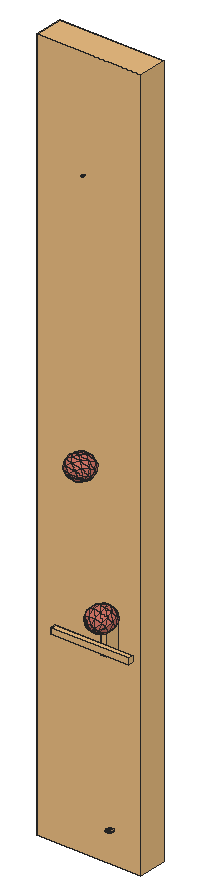
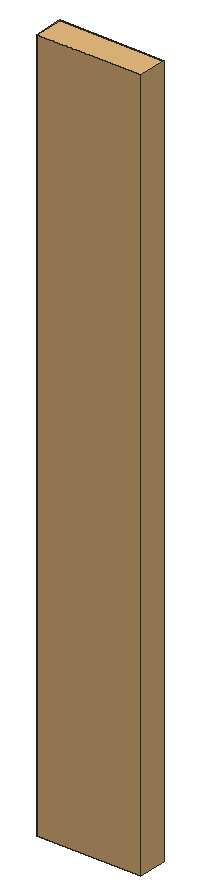
# SketchUp Ruby script. Lengths in inches.
U = 1.inch
M = Sketchup.active_model
def pt(a) = Geom::Point3d.new(a.map { |v| v * U })
def face(e, loops, mat)
  f = e.add_face(loops[0].map { |a| pt(a) })
  loops[1..].each { |l| e.add_face(l.map { |a| pt(a) }).erase! }
  f.material = f.back_material = mat if mat
  f
end
# faces: each face lists its corners as indices into pts; further lists are holes
def faces(e, pts, list, mat = nil) = list.each { |f| face(e, (f[0].is_a?(Array) ? f : [f]).map { |l| l.map { |i| pts[i] } }, mat) }
# xy, xz, yz: faces in a plane at the given z, y or x. An outline is a flat list of corners, or four numbers for a rectangle; further outlines are holes
def ring(l) = l.size == 4 ? [[l[0], l[1]], [l[2], l[1]], [l[2], l[3]], [l[0], l[3]]] : l.each_slice(2).to_a
def flat(e, list, mat, &to3) = list.each { |f| face(e, (f[0].is_a?(Array) ? f : [f]).map { |l| ring(l).map { |u, v| to3.(u, v) } }, mat) }
def xy(e, z, list, mat = nil) = flat(e, list, mat) { |x, y| [x, y, z] }
def xz(e, y, list, mat = nil) = flat(e, list, mat) { |x, z| [x, y, z] }
def yz(e, x, list, mat = nil) = flat(e, list, mat) { |y, z| [x, y, z] }
def lines(e, pts, list) = list.each { |a, b| e.add_line(pt(pts[a]), pt(pts[b])) }
# prism: a flat outline (further loops are holes) pulled along v
def prism(e, loops, v, mat = nil)
  f = face(e, loops, mat); d = Geom::Vector3d.new(v.map { |x| x * U })
  f.pushpull(f.normal.samedirection?(d) ? d.length : -d.length)
end
def box(e, o, s, mat = nil) = prism(e, [[o, [o[0] + s[0], o[1], o[2]], [o[0] + s[0], o[1] + s[1], o[2]], [o[0], o[1] + s[1], o[2]]]], [0, 0, s[2]], mat)
def at(x, y, z, deg = 0) = Geom::Transformation.translation(pt([x, y, z])) * Geom::Transformation.rotation(ORIGIN, Z_AXIS, deg.degrees)
def axes(o, x, y, z) = Geom::Transformation.new([*x, 0, *y, 0, *z, 0, *pt(o).to_a, 1])
def part(name) = M.definitions.add(name)
# library, detail: a bought-in or finely detailed component or shape, given as its bounding box
def library(name, o, s) = part(name).tap { |d| box(d.entities, o, s) }
def detail(e, o, s) = box(e.add_group.entities, o, s)
def put(e, d, t, mat = nil) = e.add_instance(d, t).tap { |i| i.material = mat if mat }
def group(e, t, mat = nil) = e.add_group.tap { |g| g.transformation = t; g.material = mat if mat }.entities
root = M.entities
M.materials.add("green").color = [174, 139, 102]
M.materials.add("vio").color = [206, 114, 100]
c1 = part("3DGeom~237_Defintion")
p = [[47.04,-55.62,-493.71],[-13.56,-317.59,-331.8],[-140.27,-151.99,-445.55],[202.73,-206.32,-387.4],[187.3,88.625,-451.96],[-121.25,109.98,-467.72],
  [-40.27,193.26,-443.62],[-229.4,54.34,-439.92],[-257.06,246.11,-316.41],[364.69,-39.76,-339.2],[242.94,242.09,-331.5],[-8.15,281.87,-374.07],
  [-226.21,-343.77,-187.29],[-324.43,-174.66,-320.41],[-335.72,41.26,-367.67],[202.73,-206.32,-387.4],[116.79,-398.1,-129.14],[-13.56,-317.59,-331.8],
  [202.73,-206.32,-387.4],[304.09,-301.74,-177.3],[364.69,-39.76,-339.2],[304.09,-301.74,-177.3],[202.73,-206.32,-387.4],[-33.49,352.06,-277.72],
  [242.94,242.09,-331.5],[-8.15,281.87,-374.07],[-33.49,352.06,-277.72],[-335.72,41.26,-367.67],[-324.43,-174.66,-320.41],[-456.1,-117.56,-151.8],
  [-335.72,41.26,-367.67],[-411.74,74.22,-270.32],[-335.72,41.26,-367.67],[-257.06,246.11,-316.41],[364.69,-39.76,-339.2],[444.36,-157.49,-135.55],
  [304.09,-301.74,-177.3],[428.9375,137.45,-200.11],[364.69,-39.76,-339.2],[428.9375,137.45,-200.11],[-13.56,-317.59,-331.8],[-67.38,-420.77,-4],
  [-226.21,-343.77,-187.29],[-13.56,-317.59,-331.8],[199.05,363.67,-164.61],[428.9375,137.45,-200.11],[242.94,242.09,-331.5],[-33.49,352.06,-277.72],
  [199.05,363.67,-164.61],[242.94,242.09,-331.5],[-324.43,-174.66,-320.41],[-226.21,-343.77,-187.29],[-378.25,-277.83,7.4],[-324.43,-174.66,-320.41],
  [-437.09,144.42,-173.96],[-257.06,246.11,-316.41],[-404.96,233.02,-104.42],[-257.06,246.11,-316.41],[-323.98,316.3,-80.32],[-257.06,246.11,-316.41],
  [-323.98,316.3,-80.32],[-215.84,371.9375,-108.12],[-257.06,246.11,-316.41],[-109.51,385.02,-180.37],[-33.49,352.06,-277.72],[-257.06,246.11,-316.41],
  [-257.06,246.11,-316.41],[-33.49,352.06,-277.72],[-500,4.02,15.09],[428.9375,137.45,-200.11],[500,-4.02,-15.09],[378.25,277.83,-7.4],
  [428.9375,137.45,-200.11],[199.05,363.67,-164.61],[428.9375,137.45,-200.11],[-226.21,-343.77,-187.29],[-199.05,-363.67,164.61],[-226.21,-343.77,-187.29],
  [-199.05,-363.67,164.61],[-378.25,-277.83,7.4],[67.38,420.77,4],[215.84,-371.9375,108.12],[323.98,-316.3,80.32],[323.98,-316.3,80.32],
  [304.09,-301.74,-177.3],[-444.36,157.49,135.55],[378.25,277.83,-7.4],[-428.9375,-137.45,200.11],[404.96,-233.02,104.42],[323.98,-316.3,80.32],
  [109.51,-385.02,180.37],[-116.78,398.1,129.14],[-304.09,301.73,177.3],[-304.09,301.73,177.3],[-323.98,316.3,-80.32],[-304.09,301.73,177.3],
  [437.09,-144.41,173.96],[456.1,117.56,151.8],[226.21,343.77,187.29],[226.21,343.77,187.29],[378.25,277.83,-7.4],[33.49,-352.06,277.72],
  [-199.05,-363.67,164.61],[-199.05,-363.67,164.61],[-242.94,-242.09,331.5],[-242.94,-242.09,331.5],[-364.69,39.76,339.2],[257.06,-246.11,316.41],
  [323.98,-316.3,80.32],[257.06,-246.11,316.41],[257.06,-246.11,316.41],[13.56,317.59,331.8],[-202.73,206.32,387.4],[-202.73,206.32,387.4],
  [-304.09,301.73,177.3],[411.74,-74.22,270.32],[324.43,174.66,320.41],[226.21,343.77,187.29],[-199.05,-363.67,164.61],[8.15,-281.86,374.07],
  [-242.94,-242.09,331.5],[-199.05,-363.67,164.61],[8.15,-281.86,374.07],[257.06,-246.11,316.41],[-202.73,206.32,387.4],[13.56,317.59,331.8],
  [324.43,174.66,320.41],[226.21,343.77,187.29],[-428.9375,-137.45,200.11],[-242.94,-242.09,331.5],[-187.3,-88.625,451.96],[-428.9375,-137.45,200.11],
  [-364.69,39.76,339.2],[335.72,-41.26,367.67],[257.06,-246.11,316.41],[8.15,-281.86,374.07],[33.49,-352.06,277.72],[257.06,-246.11,316.41],
  [40.27,-193.26,443.62],[257.06,-246.11,316.41],[121.25,-109.98,467.72],[257.06,-246.11,316.41],[229.4,-54.34,439.92],[257.06,-246.11,316.41],
  [335.72,-41.26,367.67],[257.06,-246.11,316.41],[140.27,151.99,445.55],[335.72,-41.26,367.67],[324.43,174.66,320.41],[13.56,317.59,331.8],
  [324.43,174.66,320.41],[-202.73,206.32,387.4],[13.56,317.59,331.8],[-364.69,39.76,339.2],[-47.04,55.62,493.71],[-364.69,39.76,339.2],
  [-202.73,206.32,387.4],[335.72,-41.26,367.67],[-202.73,206.32,387.4]]
faces(c1.entities,p,[[0,1,2],[0,3,1],[4,3,0],[5,0,2],[6,0,5],[6,4,0],[5,2,7],[5,7,8],
  [6,5,8],[4,9,3],[10,9,4],[11,4,6],[11,10,4],[2,12,13],[2,1,12],[7,2,13],
  [11,6,8],[7,13,14],[7,14,8],[15,16,17],[18,19,16],[20,21,22],[23,24,25],[26,11,8],
  [27,28,29],[30,29,31],[32,31,33],[34,35,36],[37,35,38],[10,39,9],[40,41,42],[43,16,41],
  [44,45,46],[47,48,49],[50,51,52],[53,52,29],[31,54,55],[54,56,57],[56,58,59],[60,61,62],
  [63,64,65],[61,63,66],[63,48,67],[31,29,68],[31,68,54],[69,70,35],[71,70,72],[73,71,74],
  [75,41,76],[77,78,79],[63,80,48],[61,80,63],[19,81,16],[19,82,81],[35,83,84],[54,68,85],
  [54,85,56],[80,86,48],[29,52,87],[29,87,68],[35,88,89],[70,88,35],[16,90,41],[16,81,90],
  [60,91,61],[61,91,80],[56,85,92],[56,93,94],[60,95,91],[70,96,88],[97,96,70],[71,97,70],
  [98,97,71],[80,99,100],[41,101,102],[41,90,101],[91,99,80],[52,103,104],[52,105,87],[68,87,106],
  [68,106,85],[81,82,107],[108,88,109],[88,96,110],[90,81,107],[95,111,91],[91,111,99],[85,106,112],
  [85,113,114],[97,115,96],[116,115,97],[117,116,97],[118,119,120],[121,101,122],[96,115,123],[95,124,111],
  [101,90,107],[125,126,127],[128,129,130],[131,130,132],[115,133,134],[116,133,115],[135,136,137],[138,135,139],
  [140,138,141],[142,140,143],[144,142,145],[146,147,148],[149,146,150],[129,135,138],[129,138,130],[151,146,152],
  [153,130,154],[155,154,156],[146,142,157],[158,154,146],[154,140,142],[154,142,146],[130,138,140],[130,140,154]],"vio")
c2 = library("3DGeom~136_Defintion",[-19.91,-529.75,-72.32],[39.82,1000,144.64])
c3 = part("3DGeom~46_Defintion")
p = [[-27.13,499.98,25.14],[-34.02,499.92,31.49],[-24.32,499.93,26.43],[-33.96,499.95,29.98],[-34.02,499.92,31.49],[-27.13,499.98,25.14],
  [-33.96,499.95,29.98],[-27.13,499.98,25.14],[-28.64,499.99,25.08],[-31.49,500,26.1],[-33.96,499.95,29.98],[-28.64,499.99,25.08],
  [-27.13,499.98,25.14],[-24.32,499.93,26.43],[-25.67,499.95,25.59],[-31.49,500,26.1],[-28.64,499.99,25.08],[-30.125,500,25.4],
  [-32.66,499.99,27.17],[-33.96,499.95,29.98],[-31.49,500,26.1],[-24.32,499.93,26.43],[-34.02,499.92,31.49],[-22.56,499.86,28.97],
  [-24.32,499.93,26.43],[-22.56,499.86,28.97],[-23.26,499.89,27.6],[-32.66,499.99,27.17],[-33.51,499.97,28.51],[-33.96,499.95,29.98],
  [-22.56,499.86,28.97],[-34.02,499.92,31.49],[-22.29,499.8,31.96],[-22.56,499.86,28.97],[-22.29,499.8,31.96],[-22.23,499.83,30.45],
  [-26.125,499.75,36.54],[-34.02,499.92,31.49],[-29.12,499.77,36.8],[-23.59,499.76,34.77],[-34.02,499.92,31.49],[-26.125,499.75,36.54],
  [-31.92,499.82,35.51],[-34.02,499.92,31.49],[-33.69,499.89,32.97],[-29.12,499.77,36.8],[-34.02,499.92,31.49],[-31.92,499.82,35.51],
  [-22.29,499.8,31.96],[-34.02,499.92,31.49],[-23.59,499.76,34.77],[-22.29,499.8,31.96],[-23.59,499.76,34.77],[-22.74,499.78,33.43],
  [-31.92,499.82,35.51],[-33.69,499.89,32.97],[-32.99,499.85,34.33],[-23.59,499.76,34.77],[-26.125,499.75,36.54],[-24.76,499.75,35.84],
  [-29.12,499.77,36.8],[-31.92,499.82,35.51],[-30.58,499.79,36.35],[-26.125,499.75,36.54],[-29.12,499.77,36.8],[-27.6,499.76,36.86],
  [-53.29,-499.72,58.02],[-51.39,-499.92,55.77],[-50.77,-499.95,55.72],[-53.29,-499.72,58.02],[-50.77,-499.95,55.72],[-53.24,-499.7,58.64],
  [-50.77,-499.95,55.72],[-49.57,-500,56.11],[-53.24,-499.7,58.64],[-50.77,-499.95,55.72],[-50.16,-499.98,55.83],[-49.57,-500,56.11],
  [-52.49,-499.84,56.33],[-51.39,-499.92,55.77],[-53.29,-499.72,58.02],[-52.49,-499.84,56.33],[-51.97,-499.88,55.98],[-51.39,-499.92,55.77],
  [-49.57,-500,56.11],[-48.72,-499.99,57.04],[-53.24,-499.7,58.64],[-49.57,-500,56.11],[-49.08,-500,56.53],[-48.72,-499.99,57.04],
  [-53.29,-499.72,58.02],[-52.91,-499.8,56.82],[-52.49,-499.84,56.33],[-53.29,-499.72,58.02],[-53.18,-499.76,57.41],[-52.91,-499.8,56.82],
  [-48.72,-499.99,57.04],[-48.46,-499.95,58.24],[-53.24,-499.7,58.64],[-48.72,-499.99,57.04],[-48.52,-499.98,57.63],[-48.46,-499.95,58.24],
  [-48.46,-499.95,58.24],[-48.85,-499.875,59.45],[-53.24,-499.7,58.64],[-48.46,-499.95,58.24],[-48.57,-499.91,58.86],[-48.85,-499.875,59.45],
  [-48.85,-499.875,59.45],[-49.78,-499.79,60.29],[-53.24,-499.7,58.64],[-49.78,-499.79,60.29],[-50.98,-499.72,60.54],[-53.24,-499.7,58.64],
  [-52.18,-499.68,60.16],[-53.03,-499.68,59.22],[-53.24,-499.7,58.64],[-50.98,-499.72,60.54],[-52.18,-499.68,60.16],[-53.24,-499.7,58.64],
  [-52.18,-499.68,60.16],[-52.68,-499.67,59.74],[-53.03,-499.68,59.22],[-48.85,-499.875,59.45],[-49.26,-499.83,59.9375],[-49.78,-499.79,60.29],
  [-50.98,-499.72,60.54],[-51.6,-499.69,60.4375],[-52.18,-499.68,60.16],[-49.78,-499.79,60.29],[-50.36,-499.75,60.49],[-50.98,-499.72,60.54]]
faces(c3.entities,p,[[0,1,2],[3,4,5],[6,7,8],[9,10,11],[12,13,14],[15,16,17],[18,19,20],[21,22,23],
  [24,25,26],[27,28,29],[30,31,32],[33,34,35],[36,37,38],[39,40,41],[42,43,44],[45,46,47],
  [48,49,50],[51,52,53],[54,55,56],[57,58,59],[60,61,62],[63,64,65],[66,67,68],[69,70,71],
  [72,73,74],[75,76,77],[78,79,80],[81,82,83],[84,85,86],[87,88,89],[90,91,92],[93,94,95],
  [96,97,98],[99,100,101],[102,103,104],[105,106,107],[108,109,110],[111,112,113],[114,115,116],[117,118,119],
  [120,121,122],[123,124,125],[126,127,128],[129,130,131]],"green")
c4 = library("3DGeom~169_Defintion",[-36.08,-38.12,-500],[72.16,76.24,1000])
c5 = part("3DGeom~170_Defintion")
p = [[22.63,21.29,-499.8],[10.94,15.58,-499.92],[15.89,19.76,-500],[22.63,21.29,-499.8],[9.12,9.86,-499.6],[10.94,15.58,-499.92],
  [22.63,21.29,-499.8],[22.56,-1.57,-498.16],[15.83,-0.04,-498.58],[22.63,21.29,-499.8],[29.3,-0.04,-497.96],[22.56,-1.57,-498.16],
  [22.63,21.29,-499.8],[15.83,-0.04,-498.58],[10.91,4.15,-499.1],[22.63,21.29,-499.8],[34.25,4.15,-498.04],[29.3,-0.04,-497.96],
  [22.63,21.29,-499.8],[10.91,4.15,-499.1],[9.12,9.86,-499.6],[22.63,21.29,-499.8],[36.08,9.86,-498.37],[34.25,4.15,-498.04],
  [22.63,21.29,-499.8],[34.29,15.58,-498.86],[36.08,9.86,-498.37],[22.63,21.29,-499.8],[29.37,19.76,-499.39],[34.29,15.58,-498.86],
  [-22.3,-38.12,487.14],[-22.89,-17.99,500],[-34.125,-33.09,489.82],[-22.3,-38.12,487.14],[-34.125,-33.09,489.82],[-29.08,-36.77,487.69],
  [-10.78,-33.09,490.89],[-22.89,-17.99,500],[-22.3,-38.12,487.14],[-10.78,-33.09,490.89],[-22.3,-38.12,487.14],[-15.6,-36.77,488.31],
  [-34.125,-33.09,489.82],[-34.42,-23.02,496.25],[-36.08,-28.06,492.96],[-34.125,-33.09,489.82],[-22.89,-17.99,500],[-34.42,-23.02,496.25],
  [-11.07,-23.02,497.32],[-22.89,-17.99,500],[-10.78,-33.09,490.89],[-11.07,-23.02,497.32],[-10.78,-33.09,490.89],[-9.12,-28.06,494.18],
  [-22.89,-17.99,500],[-29.59,-19.34,498.83],[-34.42,-23.02,496.25],[-22.89,-17.99,500],[-11.07,-23.02,497.32],[-16.11,-19.34,499.45]]
faces(c5.entities,p,[[0,1,2],[3,4,5],[6,7,8],[9,10,11],[12,13,14],[15,16,17],[18,19,20],[21,22,23],
  [24,25,26],[27,28,29],[30,31,32],[33,34,35],[36,37,38],[39,40,41],[42,43,44],[45,46,47],
  [48,49,50],[51,52,53],[54,55,56],[57,58,59]],"green")
c6 = part("3DGeom~233_Defintion")
p = [[65.95,-313.47,-334.33],[-179.28,-246.09,-369.2],[-76.8125,-70.73,-489.54],[154.6875,-161.61,-438.54],[-287.73,39.11,-409.37],[46.24,123.59,-478.71],
  [-181.17,207.39,-399.98],[261.25,6.67,-429.16],[261.25,6.67,-429.16],[156.9,284.78,-339.6],[-85.33,346.99,-279.51],[-85.33,346.99,-279.51],
  [156.9,284.78,-339.6],[293.5,-296.87,-209.87],[293.5,-296.87,-209.87],[344.74,-209.1875,-270.04],[344.74,-209.1875,-270.04],[261.25,6.67,-429.16],
  [344.74,-209.1875,-270.04],[261.25,6.67,-429.16],[406.26,-112.03,-264.62],[406.26,-112.03,-264.62],[261.25,6.67,-429.16],[357.09,146.27,-308.69],
  [261.25,6.67,-429.16],[156.9,284.78,-339.6],[357.09,146.27,-308.69],[-376.47,-112.76,-305.15],[-376.47,-112.76,-305.15],[-421.55,138.46,-219.5],
  [-287.73,39.11,-409.37],[-421.55,138.46,-219.5],[-360.03,235.62,-214.08],[-360.03,235.62,-214.08],[-181.17,207.39,-399.98],[-360.03,235.62,-214.08],
  [-304.7,316.22,-144.53],[-181.17,207.39,-399.98],[-85.33,346.99,-279.51],[18.81,-408.24,-144.44],[-233.71,-355.51,-149.9375],[-179.28,-246.09,-369.2],
  [-179.28,-246.09,-369.2],[65.95,-313.47,-334.33],[-233.71,-355.51,-149.9375],[-376.47,-112.76,-305.15],[-179.28,-246.09,-369.2],[156.9,284.78,-339.6],
  [225.52,369.67,-109.5],[156.9,284.78,-339.6],[-25.9,420.5,-80.24],[156.9,284.78,-339.6],[225.52,369.67,-109.5],[266.29,-351.58,-100.24],
  [65.95,-313.47,-334.33],[266.29,-351.58,-100.24],[65.95,-313.47,-334.33],[293.5,-296.87,-209.87],[461.59,-31.43,-195.07],[416.51,219.79,-109.42],
  [-233.71,-355.51,-149.9375],[-423.61,-207.52,-115.26],[-376.47,-112.76,-305.15],[-472.79,50.78,-159.33],[-376.47,-112.76,-305.15],[-376.47,-112.76,-305.15],
  [-421.55,138.46,-219.5],[-270.39,358.66,-29.48],[293.5,-296.87,-209.87],[344.74,-209.1875,-270.04],[442.42,-200.72,-29.18],[-421.55,138.46,-219.5],
  [-442.42,200.72,29.18],[-360.03,235.62,-214.08],[-421.55,138.46,-219.5],[-304.7,316.22,-144.53],[-360.03,235.62,-214.08],[266.29,-351.58,-100.24],
  [495.9,11.01,-80.02],[-500,-3.93,-49.7],[25.9,-420.5,80.24],[-225.52,-369.67,109.5],[-225.52,-369.67,109.5],[-233.71,-355.51,-149.9375],
  [-270.39,358.66,-29.48],[-304.7,316.22,-144.53],[270.39,-358.66,29.48],[270.39,-358.66,29.48],[266.29,-351.58,-100.24],[-225.52,-369.67,109.5],
  [-416.51,-219.79,109.42],[233.71,355.51,149.9375],[225.52,369.67,-109.5],[-18.81,408.24,144.44],[233.71,355.51,149.9375],[225.52,369.67,-109.5],
  [423.61,207.52,115.26],[270.39,-358.66,29.48],[-266.29,351.58,100.24],[500,3.93,49.7],[-495.9,-11.01,80.02],[-266.29,351.58,100.24],
  [-270.39,358.66,-29.48],[304.7,-316.22,144.53],[360.03,-235.62,214.08],[421.55,-138.46,219.5],[472.79,-50.78,159.33],[-461.59,31.43,195.07],
  [-406.26,112.03,264.62],[-344.74,209.1875,270.04],[-344.74,209.1875,270.04],[-293.5,296.87,209.87],[-293.5,296.87,209.87],[-266.29,351.58,100.24],
  [304.7,-316.22,144.53],[270.39,-358.66,29.48],[376.47,112.76,305.15],[-357.09,-146.27,308.69],[85.33,-346.99,279.51],[304.7,-316.22,144.53],
  [-293.5,296.87,209.87],[-156.9,-284.78,339.6],[-225.52,-369.67,109.5],[-156.9,-284.78,339.6],[-156.9,-284.78,339.6],[179.28,246.09,369.2],
  [179.28,246.09,369.2],[-293.5,296.87,209.87],[-65.95,313.47,334.33],[233.71,355.51,149.9375],[-65.95,313.47,334.33],[360.03,-235.62,214.08],
  [304.7,-316.22,144.53],[233.71,355.51,149.9375],[-65.95,313.47,334.33],[179.28,246.09,369.2],[287.73,-39.11,409.37],[287.73,-39.11,409.37],
  [-261.25,-6.67,429.16],[-261.25,-6.67,429.16],[-65.95,313.47,334.33],[-293.5,296.87,209.87],[-344.74,209.1875,270.04],[360.03,-235.62,214.08],
  [181.17,-207.39,399.98],[421.55,-138.46,219.5],[181.17,-207.39,399.98],[360.03,-235.62,214.08],[421.55,-138.46,219.5],[287.73,-39.11,409.37],
  [181.17,-207.39,399.98],[-154.6875,161.61,438.54],[-406.26,112.03,264.62],[-261.25,-6.67,429.16],[-406.26,112.03,264.62],[181.17,-207.39,399.98],
  [-156.9,-284.78,339.6],[85.33,-346.99,279.51],[376.47,112.76,305.15],[76.8125,70.73,489.54],[376.47,112.76,305.15],[179.28,246.09,369.2],
  [-46.24,-123.58,478.71],[-357.09,-146.27,308.69],[-156.9,-284.78,339.6],[-357.09,-146.27,308.69],[181.17,-207.39,399.98],[-156.9,-284.78,339.6],
  [181.17,-207.39,399.98]]
faces(c6.entities,p,[[0,1,2],[0,2,3],[1,4,2],[3,2,5],[2,4,6],[2,6,5],[3,5,7],[8,5,9],
  [5,6,10],[5,11,12],[13,0,3],[14,3,15],[16,3,17],[18,19,20],[21,22,23],[24,25,26],
  [1,27,4],[28,29,30],[4,31,32],[4,33,6],[34,35,36],[37,36,38],[39,40,41],[39,42,43],
  [44,45,46],[23,47,48],[49,38,50],[51,50,52],[53,39,54],[55,56,57],[21,23,58],[58,23,59],
  [23,48,59],[60,61,62],[61,63,64],[65,63,66],[38,36,67],[38,67,50],[68,69,70],[69,21,70],
  [21,58,70],[71,63,72],[73,74,72],[75,76,72],[77,68,70],[58,78,70],[58,59,78],[61,79,63],
  [63,79,72],[80,81,40],[80,40,39],[82,61,83],[84,85,72],[86,80,39],[87,39,88],[89,90,61],
  [90,79,61],[59,48,91],[92,93,94],[95,50,93],[78,59,96],[59,91,96],[97,77,70],[50,67,98],
  [50,98,93],[78,99,70],[78,96,99],[90,100,79],[79,100,72],[101,102,72],[103,97,70],[104,103,70],
  [105,104,70],[106,105,70],[99,106,70],[100,107,72],[107,108,72],[108,109,72],[110,111,72],[112,113,72],
  [114,80,115],[99,116,106],[99,96,116],[117,100,90],[117,107,100],[118,81,80],[119,118,80],[93,98,120],
  [121,90,122],[123,117,90],[118,124,81],[96,125,116],[96,91,126],[93,127,128],[129,93,130],[131,118,132],
  [133,134,135],[106,136,105],[106,116,137],[138,107,117],[139,108,107],[140,141,142],[143,144,118],[145,146,147],
  [148,149,150],[151,152,153],[151,142,154],[140,142,151],[155,156,157],[158,159,149],[160,161,159],[162,163,164],
  [162,153,165],[161,140,151],[166,162,167],[161,151,159],[149,162,168],[149,159,162],[159,153,162],[159,151,153]],"vio")
c7 = library("3DGeom~142_Defintion",[-333.55,-500,-87.71],[667.1,1000,175.42])
c8 = part("3DGeom~143_Defintion")
p = [[307.12,492.85,-37.96],[315.07,468.23,21.32],[327.57,466.68,8.76],[307.12,492.85,-37.96],[327.57,466.68,8.76],[333.55,469.6,-7.65],
  [307.12,492.85,-37.96],[299.4,473.83,26.65],[315.07,468.23,21.32],[307.12,492.85,-37.96],[333.55,469.6,-7.65],[331.42,476.19,-23.54],
  [307.12,492.85,-37.96],[284.77,481.97,23.32],[299.4,473.83,26.65],[307.12,492.85,-37.96],[331.42,476.19,-23.54],[321.75,484.71,-34.63],
  [307.12,492.85,-37.96],[275.09,490.49,12.23],[284.77,481.97,23.32],[307.12,492.85,-37.96],[272.96,497.08,-3.66],[275.09,490.49,12.23],
  [307.12,492.85,-37.96],[278.95,500,-20.08],[272.96,497.08,-3.66],[307.12,492.85,-37.96],[291.45,498.45,-32.63],[278.95,500,-20.08],
  [-307.72,-489.79,19.99],[-291.97,-496.19,23.52],[-279.25,-499.93,35.1875],[-274.79,-496.39,69.05],[-307.72,-489.79,19.99],[-279.25,-499.93,35.1875],
  [-298.8,-482.72,87.71],[-307.72,-489.79,19.99],[-274.79,-496.39,69.05],[-331.73,-476.12,38.65],[-307.72,-489.79,19.99],[-327.27,-472.59,72.51],
  [-307.72,-489.79,19.99],[-331.73,-476.12,38.65],[-322.27,-482.45,25.52],[-327.27,-472.59,72.51],[-307.72,-489.79,19.99],[-298.8,-482.72,87.71],
  [-274.79,-496.39,69.05],[-279.25,-499.93,35.1875],[-272.96,-500,51.85],[-331.73,-476.12,38.65],[-327.27,-472.59,72.51],[-333.55,-472.51,55.85],
  [-298.8,-482.72,87.71],[-274.79,-496.39,69.05],[-284.25,-490.06,82.18],[-327.27,-472.59,72.51],[-298.8,-482.72,87.71],[-314.54,-476.32,84.17]]
faces(c8.entities,p,[[0,1,2],[3,4,5],[6,7,8],[9,10,11],[12,13,14],[15,16,17],[18,19,20],[21,22,23],
  [24,25,26],[27,28,29],[30,31,32],[33,34,35],[36,37,38],[39,40,41],[42,43,44],[45,46,47],
  [48,49,50],[51,52,53],[54,55,56],[57,58,59]],"green")
g1 = group(root,at(15.3125,134.49,26.21))
put(g1,c1,axes([-1.55,0.1875,9.07],[0,0.00039,0],[0,0,-0.00039],[-0.00039,0,0]),"vio")
put(root,c2,axes([13.77,135.02,35.07],[0,0.01014,0],[0,0,-0.01014],[-0.01014,0,0]),"green")
put(root,c3,axes([14.37,134.99,34.91],[0,0.00829,0],[0,0,-0.00829],[-0.00829,0,0]),"green")
g2 = group(root,at(15.3125,134.49,26.21))
put(g2,c4,axes([-1.27,0.04,6.98],[0,0.0011,0],[0,0,-0.0011],[-0.0011,0,0]),"green")
put(g2,c5,axes([-1.27,0.04,6.98],[0,0.0011,0],[0,0,-0.0011],[-0.0011,0,0]),"green")
g3 = group(root,at(15.3125,134.49,26.21))
put(g3,c6,axes([-1.2,0.12,7.3],[0,0.00039,0],[0,0,-0.00039],[-0.00039,0,0]),"vio")
g4 = group(root,at(15.3125,134.49,26.21))
put(g4,c7,axes([-1.17,0.27,7.05],[0,0.00043,0],[0,0,-0.00043],[-0.00043,0,0]),"green")
put(g4,c8,axes([-1.17,0.27,7.05],[0,0.00043,0],[0,0,-0.00043],[-0.00043,0,0]),"green")
